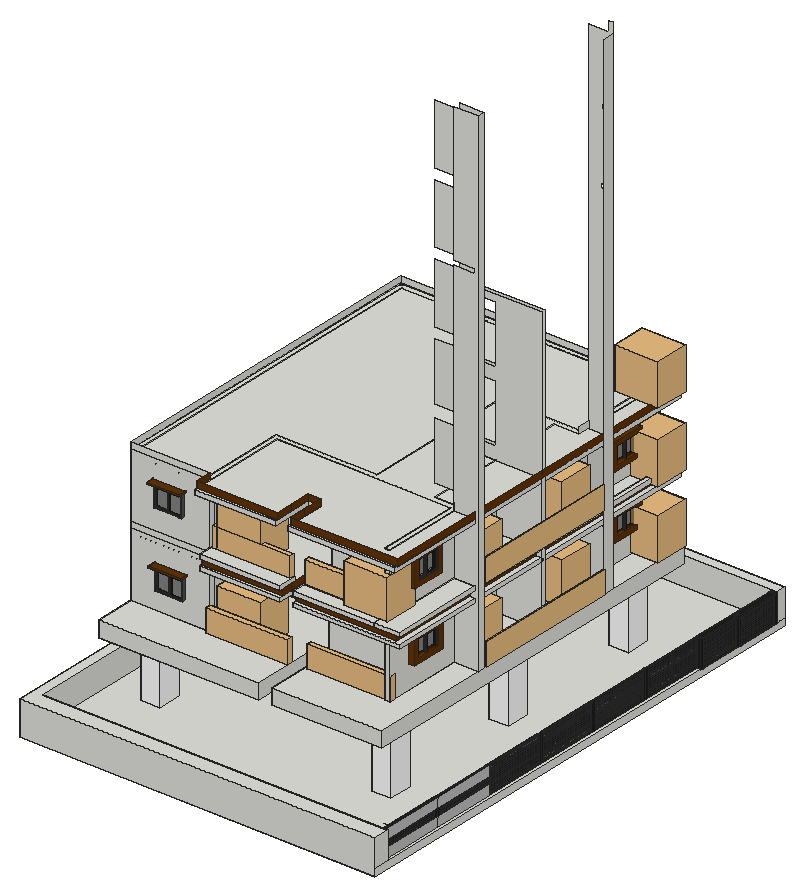
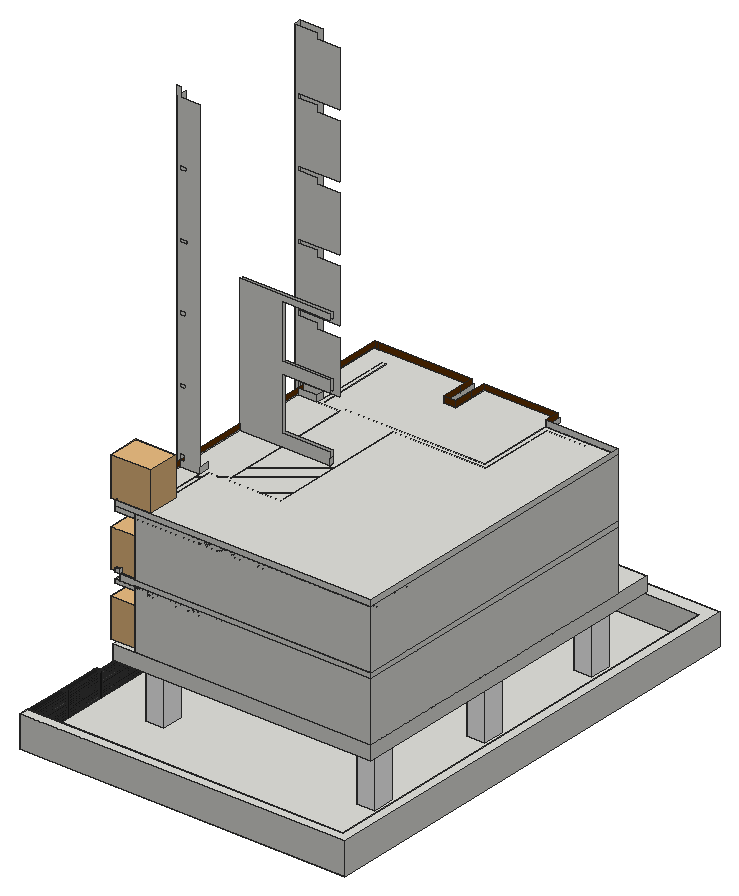
# SketchUp Ruby script. Lengths in inches.
U = 1.inch
M = Sketchup.active_model
def pt(a) = Geom::Point3d.new(a.map { |v| v * U })
def face(e, loops, mat)
  f = e.add_face(loops[0].map { |a| pt(a) })
  loops[1..].each { |l| e.add_face(l.map { |a| pt(a) }).erase! }
  f.material = f.back_material = mat if mat
  f
end
# faces: each face lists its corners as indices into pts; further lists are holes
def faces(e, pts, list, mat = nil) = list.each { |f| face(e, (f[0].is_a?(Array) ? f : [f]).map { |l| l.map { |i| pts[i] } }, mat) }
# xy, xz, yz: faces in a plane at the given z, y or x. An outline is a flat list of corners, or four numbers for a rectangle; further outlines are holes
def ring(l) = l.size == 4 ? [[l[0], l[1]], [l[2], l[1]], [l[2], l[3]], [l[0], l[3]]] : l.each_slice(2).to_a
def flat(e, list, mat, &to3) = list.each { |f| face(e, (f[0].is_a?(Array) ? f : [f]).map { |l| ring(l).map { |u, v| to3.(u, v) } }, mat) }
def xy(e, z, list, mat = nil) = flat(e, list, mat) { |x, y| [x, y, z] }
def xz(e, y, list, mat = nil) = flat(e, list, mat) { |x, z| [x, y, z] }
def yz(e, x, list, mat = nil) = flat(e, list, mat) { |y, z| [x, y, z] }
def lines(e, pts, list) = list.each { |a, b| e.add_line(pt(pts[a]), pt(pts[b])) }
# prism: a flat outline (further loops are holes) pulled along v
def prism(e, loops, v, mat = nil)
  f = face(e, loops, mat); d = Geom::Vector3d.new(v.map { |x| x * U })
  f.pushpull(f.normal.samedirection?(d) ? d.length : -d.length)
end
def box(e, o, s, mat = nil) = prism(e, [[o, [o[0] + s[0], o[1], o[2]], [o[0] + s[0], o[1] + s[1], o[2]], [o[0], o[1] + s[1], o[2]]]], [0, 0, s[2]], mat)
def at(x, y, z, deg = 0) = Geom::Transformation.translation(pt([x, y, z])) * Geom::Transformation.rotation(ORIGIN, Z_AXIS, deg.degrees)
def axes(o, x, y, z) = Geom::Transformation.new([*x, 0, *y, 0, *z, 0, *pt(o).to_a, 1])
def part(name) = M.definitions.add(name)
# library, detail: a bought-in or finely detailed component or shape, given as its bounding box
def library(name, o, s) = part(name).tap { |d| box(d.entities, o, s) }
def detail(e, o, s) = box(e.add_group.entities, o, s)
def put(e, d, t, mat = nil) = e.add_instance(d, t).tap { |i| i.material = mat if mat }
def group(e, t, mat = nil) = e.add_group.tap { |g| g.transformation = t; g.material = mat if mat }.entities
root = M.entities
M.materials.add("Color_008").color = [30, 30, 30]
M.materials.add("Glass_Tinted_Gray").color = [0, 0, 0]
M.materials["Glass_Tinted_Gray"].alpha = 0.125
M.materials.add("[0055_LightGoldenrodYellow]").color = [250, 250, 210]
M.materials.add("[0131_Silver]").color = [192, 192, 192]
M.materials.add("[0134_DimGray]").color = [105, 105, 105]
M.materials.add("[0135_DarkGray]").color = [81, 81, 81]
M.materials.add("[Color C08]").color = [102, 51, 0]
M.materials.add("[Color M00]").color = [255, 255, 255]
M.materials.add("[Mirror 02]").color = [229, 229, 229]
M.materials.add("[Terrazzo Light Blue]").color = [196, 214, 227]
c1 = part("Gate infill panel")
box(c1.entities,[0,0,-9.84],[39.64,0.39,36.58])
c2 = part("Gate frame stile")
box(c2.entities,[0,0,0],[1.9,0.97,93.54])
c3 = part("Gate slat \#1")
box(c3.entities,[2.95,0,-2.03],[0.99,0.97,40.94])
c4 = part("Gate slat")
box(c4.entities,[0,0,-2.03],[1.97,0.97,40.94])
c5 = part("Slatted gate leaf")
p = [[42.85,0.97,43.31],[42.85,0.97,44.29]]
lines(c5.entities,p,[[0,1]])
put(c5.entities,c2,axes([87.6,0,0],[1,0,0],[0,1,0],[0,0,0.92593]),"Color_008")
put(c5.entities,c2,axes([0,0,0],[1,0,0],[0,1,0],[0,0,0.92593]),"Color_008")
put(c5.entities,c2,axes([42.85,0,0],[1,0,0],[0,1,0],[0,0,0.92593]),"Color_008")
put(c5.entities,c2,axes([44.75,0,0],[1,0,0],[0,1,0],[0,0,0.92593]),"Color_008")
put(c5.entities,c3,axes([3.9375,0,6.89],[0,0,-1],[0,1,0],[1,0,0]),"[0134_DimGray]")
put(c5.entities,c3,axes([48.6875,0,6.89],[0,0,-1],[0,1,0],[1,0,0]),"[0134_DimGray]")
put(c5.entities,c3,axes([48.6875,0,11.71],[0,0,-1],[0,1,0],[1,0,0]),"[0134_DimGray]")
put(c5.entities,c4,axes([48.6875,0,6.79],[0,0,-1],[0,1,0],[1,0,0]),"Color_008")
put(c5.entities,c4,axes([3.9375,0,6.79],[0,0,-1],[0,1,0],[1,0,0]),"Color_008")
put(c5.entities,c3,axes([3.9375,0,11.71],[0,0,-1],[0,1,0],[1,0,0]),"[0134_DimGray]")
put(c5.entities,c4,axes([3.9375,0,11.61],[0,0,-1],[0,1,0],[1,0,0]),"Color_008")
put(c5.entities,c3,axes([3.9375,0,16.54],[0,0,-1],[0,1,0],[1,0,0]),"[0134_DimGray]")
put(c5.entities,c3,axes([48.6875,0,16.54],[0,0,-1],[0,1,0],[1,0,0]),"[0134_DimGray]")
put(c5.entities,c3,axes([48.6875,0,21.36],[0,0,-1],[0,1,0],[1,0,0]),"[0134_DimGray]")
put(c5.entities,c4,axes([48.6875,0,11.61],[0,0,-1],[0,1,0],[1,0,0]),"Color_008")
put(c5.entities,c3,axes([3.9375,0,21.36],[0,0,-1],[0,1,0],[1,0,0]),"[0134_DimGray]")
put(c5.entities,c4,axes([3.9375,0,26.08],[0,0,-1],[0,1,0],[1,0,0]),"Color_008")
put(c5.entities,c3,axes([3.9375,0,31],[0,0,-1],[0,1,0],[1,0,0]),"[0134_DimGray]")
put(c5.entities,c3,axes([3.9375,0,26.18],[0,0,-1],[0,1,0],[1,0,0]),"[0134_DimGray]")
put(c5.entities,c4,axes([48.6875,0,30.91],[0,0,-1],[0,1,0],[1,0,0]),"Color_008")
put(c5.entities,c4,axes([48.6875,0,21.26],[0,0,-1],[0,1,0],[1,0,0]),"Color_008")
put(c5.entities,c4,axes([3.9375,0,21.26],[0,0,-1],[0,1,0],[1,0,0]),"Color_008")
put(c5.entities,c4,axes([48.6875,0,41.7],[0,0,-1],[0,1,0],[1,0,0]),"Color_008")
put(c5.entities,c4,axes([48.6875,0,26.08],[0,0,-1],[0,1,0],[1,0,0]),"Color_008")
put(c5.entities,c4,axes([3.9375,0,35.73],[0,0,-1],[0,1,0],[1,0,0]),"Color_008")
put(c5.entities,c4,axes([3.9375,0,41.7],[0,0,-1],[0,1,0],[1,0,0]),"Color_008")
put(c5.entities,c4,axes([48.6875,0,35.73],[0,0,-1],[0,1,0],[1,0,0]),"Color_008")
put(c5.entities,c3,axes([48.6875,0,31],[0,0,-1],[0,1,0],[1,0,0]),"[0134_DimGray]")
put(c5.entities,c3,axes([48.6875,0,26.18],[0,0,-1],[0,1,0],[1,0,0]),"[0134_DimGray]")
put(c5.entities,c3,axes([3.9375,0,67.42],[0,0,-1],[0,1,0],[1,0,0]),"[0134_DimGray]")
put(c5.entities,c4,axes([48.6875,0,57.68],[0,0,-1],[0,1,0],[1,0,0]),"Color_008")
put(c5.entities,c4,axes([48.6875,0,52.85],[0,0,-1],[0,1,0],[1,0,0]),"Color_008")
put(c5.entities,c4,axes([3.9375,0,30.91],[0,0,-1],[0,1,0],[1,0,0]),"Color_008")
put(c5.entities,c3,axes([48.6875,0,57.78],[0,0,-1],[0,1,0],[1,0,0]),"[0134_DimGray]")
put(c5.entities,c4,axes([48.6875,0,62.5],[0,0,-1],[0,1,0],[1,0,0]),"Color_008")
put(c5.entities,c4,axes([3.9375,0,57.68],[0,0,-1],[0,1,0],[1,0,0]),"Color_008")
put(c5.entities,c4,axes([3.9375,0,62.5],[0,0,-1],[0,1,0],[1,0,0]),"Color_008")
put(c5.entities,c3,axes([48.6875,0,67.42],[0,0,-1],[0,1,0],[1,0,0]),"[0134_DimGray]")
put(c5.entities,c3,axes([48.6875,0,62.6],[0,0,-1],[0,1,0],[1,0,0]),"[0134_DimGray]")
put(c5.entities,c3,axes([3.9375,0,62.6],[0,0,-1],[0,1,0],[1,0,0]),"[0134_DimGray]")
put(c5.entities,c4,axes([48.6875,0,46.88],[0,0,-1],[0,1,0],[1,0,0]),"Color_008")
put(c5.entities,c4,axes([3.9375,0,52.85],[0,0,-1],[0,1,0],[1,0,0]),"Color_008")
put(c5.entities,c4,axes([3.9375,0,46.88],[0,0,-1],[0,1,0],[1,0,0]),"Color_008")
put(c5.entities,c3,axes([3.9375,0,57.78],[0,0,-1],[0,1,0],[1,0,0]),"[0134_DimGray]")
put(c5.entities,c4,axes([48.6875,0,16.4375],[0,0,-1],[0,1,0],[1,0,0]),"Color_008")
put(c5.entities,c4,axes([3.9375,0,16.4375],[0,0,-1],[0,1,0],[1,0,0]),"Color_008")
put(c5.entities,c4,axes([48.6875,0,1.97],[0,0,-1],[0,1,0],[1,0,0]),"Color_008")
put(c5.entities,c4,axes([3.9375,0,1.97],[0,0,-1],[0,1,0],[1,0,0]),"Color_008")
put(c5.entities,c3,axes([3.9375,0,81.89],[0,0,-1],[0,1,0],[1,0,0]),"[0134_DimGray]")
put(c5.entities,c4,axes([48.6875,0,72.15],[0,0,-1],[0,1,0],[1,0,0]),"Color_008")
put(c5.entities,c4,axes([48.6875,0,67.32],[0,0,-1],[0,1,0],[1,0,0]),"Color_008")
put(c5.entities,c3,axes([48.6875,0,72.24],[0,0,-1],[0,1,0],[1,0,0]),"[0134_DimGray]")
put(c5.entities,c3,axes([3.9375,0,72.24],[0,0,-1],[0,1,0],[1,0,0]),"[0134_DimGray]")
put(c5.entities,c4,axes([3.9375,0,72.15],[0,0,-1],[0,1,0],[1,0,0]),"Color_008")
put(c5.entities,c3,axes([3.9375,0,77.07],[0,0,-1],[0,1,0],[1,0,0]),"[0134_DimGray]")
put(c5.entities,c3,axes([48.6875,0,81.89],[0,0,-1],[0,1,0],[1,0,0]),"[0134_DimGray]")
put(c5.entities,c4,axes([3.9375,0,76.97],[0,0,-1],[0,1,0],[1,0,0]),"Color_008")
put(c5.entities,c4,axes([48.6875,0,76.97],[0,0,-1],[0,1,0],[1,0,0]),"Color_008")
put(c5.entities,c3,axes([48.6875,0,77.07],[0,0,-1],[0,1,0],[1,0,0]),"[0134_DimGray]")
put(c5.entities,c4,axes([3.9375,0,67.32],[0,0,-1],[0,1,0],[1,0,0]),"Color_008")
put(c5.entities,c4,axes([48.6875,0,86.61],[0,0,-1],[0,1,0],[1,0,0]),"Color_008")
put(c5.entities,c4,axes([48.6875,0,81.79],[0,0,-1],[0,1,0],[1,0,0]),"Color_008")
put(c5.entities,c3,axes([3.9375,0,86.71],[0,0,-1],[0,1,0],[1,0,0]),"[0134_DimGray]")
put(c5.entities,c3,axes([48.6875,0,86.71],[0,0,-1],[0,1,0],[1,0,0]),"[0134_DimGray]")
put(c5.entities,c4,axes([3.9375,0,86.61],[0,0,-1],[0,1,0],[1,0,0]),"Color_008")
put(c5.entities,c4,axes([3.9375,0,81.79],[0,0,-1],[0,1,0],[1,0,0]),"Color_008")
put(c5.entities,c3,axes([48.6875,0,35.83],[0,0,-1],[0,1,0],[1,0,0]),"[0134_DimGray]")
put(c5.entities,c3,axes([3.9375,0,35.83],[0,0,-1],[0,1,0],[1,0,0]),"[0134_DimGray]")
c6 = part("Gate infill panel \#1")
box(c6.entities,[0,0,-1.97],[52.81,0.39,23.62])
c7 = part("Porton casa")
put(c7.entities,c1,axes([2026.52,648.38,306.58],[0,-3.00253,0],[2.8696,0,0],[0,0,0.48432]),"[0131_Silver]")
put(c7.entities,c1,axes([2026.52,767.39,338.47],[0,-3.00253,0],[2.8696,0,0],[0,0,0.48432]),"[0131_Silver]")
put(c7.entities,c5,axes([2023.74,772.67,300.63],[0,-2.77742,0],[2.8696,0,0],[0,0,0.6]),"[0055_LightGoldenrodYellow]")
put(c7.entities,c1,axes([2026.52,767.39,306.58],[0,-3.00253,0],[2.8696,0,0],[0,0,0.48432]),"[0131_Silver]")
put(c7.entities,c6,axes([2022.61,772.67,320.71],[0,-2.3537,0],[2.8696,0,0],[0,0,0.6]),"Color_008")
put(c7.entities,c1,axes([2026.52,648.38,338.47],[0,-3.00253,0],[2.8696,0,0],[0,0,0.48432]),"[0131_Silver]")
put(c7.entities,c6,axes([2022.61,648.38,320.71],[0,-2.3537,0],[2.8696,0,0],[0,0,0.6]),"Color_008")
put(c7.entities,c5,axes([2023.74,1012.92,300.63],[0,-2.77742,0],[2.8696,0,0],[0,0,0.6]),"[0055_LightGoldenrodYellow]")
put(c7.entities,c5,axes([2023.74,1256.22,300.63],[0,-2.77742,0],[2.8696,0,0],[0,0,0.6]),"[0055_LightGoldenrodYellow]")
put(c7.entities,c5,axes([2023.74,1426.375,300.63],[0,-1.96025,0],[10.8312,0,0],[0,0,0.6]),"[0055_LightGoldenrodYellow]")
c8 = part("Group\#10")
box(c8.entities,[49.375,41.9375,0],[35.875,43.3125,120],"[Color M00]")
c9 = library("Wagner Glass Railing",[9.08,102.375,1.53],[2.51,145.5,42.05])
c10 = library("Round Planter with Plant",[-35.48,-39.77,0],[80.62,63.55,77.875])
c11 = part("PENTEK_RP Fineline 50S_Sliding_DoorCase_E1")
box(c11.entities,[0,0,0],[1.51,3.66,99.27],"[0135_DarkGray]")
c12 = part("PENTEK_RP Fineline 50S_SlidingDooe_Case_E2")
box(c12.entities,[0,0,0],[96.25,3.66,1.51],"[0135_DarkGray]")
c13 = part("pentek_RP Fineline 50S_SlidingDoor_Case")
put(c13.entities,c11,at(97.76,0,0))
put(c13.entities,c12,at(1.51,0,0))
put(c13.entities,c11,at(0,0,0))
put(c13.entities,c12,at(1.51,0,97.76))
c14 = part("PENTEK_RP Fineline 50S_SlidingDoor_GlazingBead_2")
box(c14.entities,[0,0,0],[0.56,0.59,94.39],"[0135_DarkGray]")
c15 = part("PENTEK_RP Fineline 50S_SlidingDoor_Glass")
box(c15.entities,[0,0,0],[46.58,0.16,94.39],"Glass_Tinted_Gray")
c16 = part("PENTEK_RP Fineline 50S_SlidingDoor_GlazingBead")
box(c16.entities,[0,0,0],[45.47,0.59,0.56],"[0135_DarkGray]")
c17 = part("PENTEK_RP Fineline 50S_SlidingDoor_Leaf_E1")
xy(c17.entities,0,[[0,0,0.93,1.97],[0.93,1.57,1.49,1.97]],"[0135_DarkGray]")
xy(c17.entities,96.25,[[0,0,0.93,0,0.93,1.57,1.49,1.57,1.49,1.97,0,1.97]],"[0135_DarkGray]")
xz(c17.entities,0,[[0,0,0.93,96.25]],"[0135_DarkGray]")
xz(c17.entities,1.57,[[0.93,0,1.49,95.32],[0.93,95.32,1.49,96.25]],"[0135_DarkGray]")
xz(c17.entities,1.97,[[0,0,1.49,96.25]],"[0135_DarkGray]")
yz(c17.entities,0,[[0,0,1.97,96.25]],"[0135_DarkGray]")
yz(c17.entities,0.93,[[0,0,1.57,0.93],[0,0.93,1.57,95.32],[0,95.32,1.57,96.25]],"[0135_DarkGray]")
yz(c17.entities,1.49,[[1.57,0,1.97,95.32],[1.57,95.32,1.97,96.25]],"[0135_DarkGray]")
c18 = part("PENTEK_RP Fineline 50S_SlidingDoor_Leaf_E2")
xy(c18.entities,0,[[0,0,0,1.57,0.56,1.57,0.56,1.97,46.02,1.97,46.02,1.57,46.58,1.57,46.58,0]],"[0135_DarkGray]")
xy(c18.entities,0.93,[[0,0,46.58,1.57]],"[0135_DarkGray]")
xy(c18.entities,1.49,[[0.56,1.57,46.02,1.97]],"[0135_DarkGray]")
xz(c18.entities,0,[[0,0,46.58,0.93]],"[0135_DarkGray]")
xz(c18.entities,1.57,[[0,0,0.56,0.93],[46.02,0,46.58,0.93],[0.56,0.93,46.02,1.49]],"[0135_DarkGray]")
xz(c18.entities,1.97,[[0.56,0,46.02,1.49]],"[0135_DarkGray]")
yz(c18.entities,0,[[0,0,1.57,0.93]],"[0135_DarkGray]")
yz(c18.entities,0.56,[[1.57,0,1.97,0.93],[1.57,0.93,1.97,1.49]],"[0135_DarkGray]")
yz(c18.entities,46.02,[[1.57,0,1.97,0.93],[1.57,0.93,1.97,1.49]],"[0135_DarkGray]")
yz(c18.entities,46.58,[[0,0,1.57,0.93]],"[0135_DarkGray]")
c19 = part("PENTEK_RP Fineline S_SlidingDoor_Leaf1")
put(c19.entities,c14,at(0.93,0,0.93))
put(c19.entities,c14,at(46.96,0,0.93))
put(c19.entities,c15,at(1.49,1.42,0.93))
put(c19.entities,c16,at(1.49,0,0.93))
put(c19.entities,c15,at(1.49,0.59,0.93),"[Terrazzo Light Blue]")
put(c19.entities,c17,at(0,0,0))
put(c19.entities,c17,axes([48.44,0,0],[-1,0,0],[0,1,0],[0,0,1]))
put(c19.entities,c18,axes([0.93,0,96.25],[1,0,0],[0,1,0],[0,0,-1]))
put(c19.entities,c18,at(0.93,0,0))
put(c19.entities,c16,at(1.49,0,94.77))
c20 = part("PENTEK_RP Fineline 50S_SlidingDoor_Leaf2")
put(c20.entities,c15,at(1.49,1.42,0.93))
put(c20.entities,c16,at(1.49,0,94.77))
put(c20.entities,c14,at(46.96,0,0.93))
put(c20.entities,c15,at(1.49,0.59,0.93),"[Mirror 02]")
put(c20.entities,c14,at(0.93,0,0.93))
put(c20.entities,c17,at(0,0,0))
put(c20.entities,c17,axes([48.44,0,0],[-1,0,0],[0,1,0],[0,0,1]))
put(c20.entities,c16,at(1.49,0,0.93))
put(c20.entities,c18,axes([0.93,0,96.25],[1,0,0],[0,1,0],[0,0,-1]))
put(c20.entities,c18,at(0.93,0,0))
c21 = part("PENTEK - Slimmest Steel Sliding Door / Window\#1")
put(c21.entities,c13,at(0,-1.88,-0.09))
put(c21.entities,c19,at(1.51,-2.27,1.42))
put(c21.entities,c20,at(49.32,-0.3,1.42))
c22 = part("Group\#9")
box(c22.entities,[0,0,0],[60.1875,3.0625,15.3125])
xy(root,-162.0625,[[0,0,659.75,950.625]])
xy(root,-149.5,[[19.4375,28.625,659.75,931.79]])
xy(root,-98,[[0,0,659.75,0,659.75,28.625,19.4375,28.625,19.4375,931.79,659.75,931.79,659.75,950.625,0,950.625]])
xy(root,0,[[53.0625,117.84,350.31,117.84,350.31,232.22,374.31,232.22,374.31,117.84,577.93,117.84,577.93,191.22,578.3125,191.22,578.3125,341.375,533.0625,341.375,533.0625,191.22,524.0625,191.22,524.0625,241.82,381.04,241.82,381.04,346.01,200.56,346.01,200.56,191.22,53.0625,191.22],[53.0625,191.22,200.56,191.22,200.56,346.01,381.04,346.01,381.04,241.82,524.0625,241.82,524.0625,192.09,533.0625,192.09,533.0625,355.01,486.8125,355.01,486.8125,495.28,388.3125,495.28,388.3125,502.74,486.8125,502.74,486.8125,631.35,533.0625,631.35,533.0625,638.86,524.0625,640.35,379.3125,640.35,379.3125,355.01,191.56,355.01,191.56,200.22,62.0625,200.22,62.0625,809.84,524.0625,809.84,524.0625,640.35,533.0625,638.86,533.0625,818.16,53.0625,818.16],[524.0625,191.22,533.0625,192.09],[62.0625,200.22,191.56,200.22,191.56,355.01,379.3125,355.01,379.3125,640.35,524.0625,640.35,524.0625,809.84,62.0625,809.84],[486.8125,355.01,578.3125,495.28],
  [572.25,495.28,578.3125,502.74],[486.8125,502.74,578.3125,631.35],[533.0625,631.35,578.3125,631.35,533.0625,638.86],[578.3125,631.35,578.3125,653.47,533.0625,653.47,533.0625,638.86],[533.0625,653.47,578.3125,818.16]])
xy(root,44.43,[[533.0625,234.1,545.1875,299.28],[533.0625,696.28,545.1875,761.47]],"[Color C08]")
xy(root,52.48,[[533.0625,242.15,545.1875,291.23],[533.0625,704.34,545.1875,753.42]],"[Color C08]")
xy(root,85.5625,[[533.0625,242.15,545.1875,291.23],[533.0625,704.34,545.1875,753.42]])
xy(root,93.62,[[533.0625,234.1,545.1875,299.28],[533.0625,696.28,545.1875,761.47]],"[Color C08]")
xy(root,112.625,[[381.04,241.82,524.0625,346.01]])
xy(root,120,[[[53.0625,191.22,200.56,191.22,200.56,346.01,524.0625,346.01,524.0625,191.22,533.0625,191.22,533.0625,355.01,486.8125,355.01,486.8125,495.28,388.3125,495.28,388.3125,502.74,486.8125,502.74,486.8125,631.35,533.0625,631.35,533.0625,818.16,53.0625,818.16],[62.0625,200.22,62.0625,809.84,524.0625,809.84,524.0625,640.35,379.3125,640.35,379.3125,355.01,191.56,355.01,191.56,200.22]]])
xy(root,132,[[200.56,165.97,350.31,191.22],[374.31,165.97,524.0625,191.22],[524.25,165.97,524.25,191.22,533.0625,191.22,533.0625,341.375,572.25,341.375,572.25,165.97],[[53.0625,191.22,200.56,191.22,200.56,346.01,389.59,346.01,389.59,237.76,524.0625,237.76,524.0625,191.22,533.0625,191.22,533.0625,355.01,486.8125,355.01,486.8125,495.28,388.3125,495.28,388.3125,502.74,486.8125,502.74,486.8125,631.35,533.0625,631.35,533.0625,818.16,53.0625,818.16],[62.0625,200.22,62.0625,809.84,524.0625,809.84,524.0625,640.35,379.3125,640.35,379.3125,355.01,191.56,355.01,191.56,200.22]],[62.0625,200.22,191.56,200.22,191.56,355.01,379.3125,355.01,379.3125,640.35,524.0625,640.35,524.0625,809.84,62.0625,809.84],
  [200.56,200.22,350.31,200.22,350.31,232.22,374.31,232.22,374.31,200.22,524.0625,200.22,524.0625,237.76,389.59,237.76,389.59,346.01,200.56,346.01],[486.8125,355.01,560.01,355.01,560.01,631.35,486.8125,631.35,486.8125,502.74,388.3125,502.74,388.3125,495.28,486.8125,495.28],[533.0625,641.54,572.25,641.54,572.25,653.47,563.82,653.47,563.82,818.16,533.0625,818.16]])
xy(root,139.375,[[200.56,165.97,350.31,200.22],[374.31,165.97,524.0625,200.22]])
xy(root,139.6875,[[524.25,165.97,572.25,165.97,572.25,341.375,533.0625,341.375,533.0625,191.22,524.25,191.22]])
xy(root,140.1875,[[560.01,355.01,572.25,631.35],[563.82,653.47,572.25,818.16]])
xy(root,163.74,[[533.0625,696.28,545.1875,761.47]],"[Color C08]")
xy(root,171.8,[[533.0625,704.34,545.1875,753.42]],"[Color C08]")
xy(root,171.99,[[533.0625,236.27,545.1875,298.83]],"[Color C08]")
xy(root,180.05,[[533.0625,244.32,545.1875,290.77]])
xy(root,204.875,[[533.0625,704.34,545.1875,753.42]])
xy(root,212.93,[[533.0625,696.28,545.1875,761.47]],"[Color C08]")
xy(root,217.25,[[533.0625,244.32,545.1875,290.77]],"[Color C08]")
xy(root,225.3,[[533.0625,236.27,545.1875,298.83]],"[Color C08]")
xy(root,243.8125,[[389.59,237.76,524.0625,346.01]])
xy(root,252,[[562.5625,155.07,572.25,162],[[53.0625,191.22,200.56,191.22,200.56,346.01,524.0625,346.01,524.0625,191.22,533.0625,191.22,533.0625,355.01,486.8125,355.01,486.8125,495.28,388.3125,495.28,388.3125,502.74,486.8125,502.74,486.8125,631.35,533.0625,631.35,533.0625,818.16,53.0625,818.16],[62.0625,200.22,62.0625,809.84,524.0625,809.84,524.0625,640.35,379.3125,640.35,379.3125,355.01,191.56,355.01,191.56,200.22]]])
xz(root,0,[[0,-162.0625,659.75,-98]])
xz(root,28.625,[[19.4375,-149.5,659.75,-98]])
xz(root,165.97,[[200.56,132,350.31,139.375],[374.31,132,524.0625,139.375],[524.25,132,572.25,139.6875]])
xz(root,191.22,[[53.0625,0,200.56,120],[524.0625,0,533.0625,120],[53.0625,132,200.56,252],[374.31,132,524.0625,139.375],[524.0625,132,524.25,132,524.25,139.6875,533.0625,139.6875,533.0625,252,524.0625,252],
  [524.25,132,533.0625,139.6875]])
xz(root,200.22,[[62.0625,0,191.56,120],[62.0625,132,191.56,252],[200.56,132,350.31,139.375],[374.31,132,524.0625,139.375]])
xz(root,234.1,[[533.0625,44.43,545.1875,93.62]],"[Color C08]")
xz(root,236.27,[[533.0625,171.99,545.1875,225.3]],"[Color C08]")
xz(root,237.76,[[389.59,132,524.0625,243.8125]])
xz(root,241.82,[[381.04,0,524.0625,112.625]])
xz(root,242.15,[[533.0625,52.48,545.1875,85.5625]],"[Color C08]")
xz(root,244.32,[[533.0625,180.05,545.1875,217.25]],"[Color C08]")
xz(root,290.77,[[533.0625,180.05,545.1875,217.25]],"[Color C08]")
xz(root,291.23,[[533.0625,52.48,545.1875,85.5625]],"[Color C08]")
xz(root,298.83,[[533.0625,171.99,545.1875,225.3]],"[Color C08]")
xz(root,299.28,[[533.0625,44.43,545.1875,93.62]],"[Color C08]")
xz(root,341.375,[[533.0625,0,578.3125,0,578.3125,924,533.0625,924,533.0625,668.1875,572.25,668.1875,572.25,660,533.0625,660,533.0625,139.6875,572.25,139.6875,572.25,132,533.0625,132],[533.0625,132,572.25,139.6875]])
xz(root,346.01,[[200.56,0,381.04,0,381.04,112.625,524.0625,112.625,524.0625,120,200.56,120],[200.56,132,389.59,132,389.59,243.8125,524.0625,243.8125,524.0625,252,200.56,252]])
xz(root,355.01,[[191.56,0,379.3125,120],[486.8125,0,486.8125,120,533.0625,120,533.0625,132,486.8125,132,486.8125,252,533.0625,252,533.0625,264,572.25,264,572.25,276.5625,486.8125,276.5625,486.8125,384,533.0625,384,533.0625,396,572.25,396,572.25,407.125,486.8125,407.125,486.8125,516,533.0625,516,533.0625,528,572.25,528,572.25,535.4375,486.8125,535.4375,486.8125,648,533.0625,648,533.0625,660,572.25,660,572.25,668.1875,486.8125,668.1875,486.8125,780,533.0625,780,533.0625,792,572.25,792,572.25,800.1875,486.8125,800.1875,486.8125,912,533.0625,912,533.0625,924,578.3125,924,578.3125,0],[191.56,132,379.3125,252],[560.01,132,572.25,140.1875]])
xz(root,495.28,[[388.3125,0,486.8125,120],[486.8125,0,572.25,0,572.25,528,388.3125,528,388.3125,516,486.8125,516,486.8125,407.125,388.3125,407.125,388.3125,384,486.8125,384,486.8125,276.5625,388.3125,276.5625,388.3125,252,486.8125,252,486.8125,132,388.3125,132,388.3125,120,486.8125,120],[388.3125,132,486.8125,252]])
xz(root,502.74,[[388.3125,0,486.8125,120],[486.8125,0,486.8125,120,388.3125,120,388.3125,132,486.8125,132,486.8125,252,388.3125,252,388.3125,276.5625,486.8125,276.5625,486.8125,384,388.3125,384,388.3125,407.125,486.8125,407.125,486.8125,516,388.3125,516,388.3125,528,572.25,528,572.25,0],[388.3125,132,486.8125,252]])
xz(root,631.35,[[560.01,132,572.25,140.1875]])
xz(root,640.35,[[379.3125,0,524.0625,120],[379.3125,132,524.0625,252]])
xz(root,653.47,[[[533.0625,0,578.3125,0,578.3125,943.375,570.58,943.375,570.58,924,533.0625,924],[555.82,660,572.25,668.1875],[562.82,264,572.25,276.5625],[557.85,792,572.25,800.1875],[559.99,396,572.25,404.1875],[561.5,528,572.25,536.1875],[563.82,132,572.25,140.1875]],[563.82,132,572.25,140.1875]])
xz(root,696.28,[[533.0625,44.43,545.1875,93.62],[533.0625,163.74,545.1875,212.93]],"[Color C08]")
xz(root,704.34,[[533.0625,52.48,545.1875,85.5625],[533.0625,171.8,545.1875,204.875]],"[Color C08]")
xz(root,753.42,[[533.0625,52.48,545.1875,85.5625],[533.0625,171.8,545.1875,204.875]],"[Color C08]")
xz(root,761.47,[[533.0625,44.43,545.1875,93.62],[533.0625,163.74,545.1875,212.93]],"[Color C08]")
xz(root,809.84,[[62.0625,0,524.0625,120],[62.0625,132,524.0625,252]])
xz(root,818.16,[[53.0625,0,533.0625,120],[53.0625,132,533.0625,252],[563.82,132,572.25,140.1875]])
xz(root,931.79,[[19.4375,-149.5,659.75,-98]])
xz(root,950.625,[[0,-162.0625,659.75,-98]])
yz(root,0,[[0,-162.0625,950.625,-98]])
yz(root,19.4375,[[28.625,-149.5,931.79,-98]])
yz(root,53.0625,[[191.22,0,818.16,120],[191.22,132,818.16,252]])
yz(root,62.0625,[[200.22,0,809.84,120],[200.22,132,809.84,252]])
yz(root,191.56,[[200.22,0,355.01,120],[200.22,132,355.01,252]])
yz(root,200.56,[[191.22,0,200.22,120],[200.22,0,346.01,120],[165.97,132,191.22,139.375],[191.22,132,200.22,139.375],[200.22,132,346.01,252],
  [191.22,139.375,200.22,252]])
yz(root,350.31,[[165.97,132,200.22,139.375]])
yz(root,374.31,[[165.97,132,191.22,139.375],[191.22,132,200.22,139.375]])
yz(root,379.3125,[[355.01,0,640.35,120],[355.01,132,640.35,252]])
yz(root,381.04,[[241.82,0,346.01,112.625]])
yz(root,388.3125,[[495.28,0,502.74,120],[495.28,120,502.74,132],[495.28,132,502.74,252],[495.28,252,502.74,264]])
yz(root,389.59,[[237.76,132,346.01,243.8125]])
yz(root,486.8125,[[355.01,0,495.28,120],[502.74,0,631.35,120],[355.01,132,495.28,252],[502.74,132,631.35,252]])
yz(root,524.0625,[[191.22,0,200.22,120],[200.22,0,200.22,120,346.01,120,346.01,112.625,241.82,112.625,241.82,0],[640.35,0,809.84,120],[165.97,132,191.22,139.375],[191.22,132,200.22,139.375],
  [200.22,132,200.22,252,346.01,252,346.01,243.8125,237.76,243.8125,237.76,132],[640.35,132,809.84,252],[191.22,139.375,200.22,252]])
yz(root,524.25,[[165.97,132,191.22,139.6875]])
yz(root,533.0625,[[[191.22,0,341.375,120],[234.1,44.43,299.28,93.62]],[[653.47,0,818.16,120],[696.28,44.43,761.47,93.62]],[242.15,52.48,291.23,85.5625],[704.34,52.48,753.42,85.5625],[341.375,120,355.01,132],
  [631.35,120,653.47,132],[191.22,132,341.375,139.6875],[[653.47,132,818.16,252],[696.28,163.74,761.47,212.93]],[[191.22,139.6875,341.375,252],[236.27,171.99,298.83,225.3]],[704.34,171.8,753.42,204.875],
  [244.32,180.05,290.77,217.25],[341.375,252,355.01,264],[631.35,252,653.47,264]])
yz(root,545.1875,[[[234.1,44.43,299.28,93.62],[242.15,52.48,291.23,85.5625]],[[696.28,44.43,761.47,93.62],[704.34,52.48,753.42,85.5625]],[[696.28,163.74,761.47,212.93],[704.34,171.8,753.42,204.875]],[[236.27,171.99,298.83,225.3],[244.32,180.05,290.77,217.25]]],"[Color C08]")
yz(root,560.01,[[355.01,132,495.28,140.1875],[495.28,132,502.74,140.1875],[502.74,132,631.35,140.1875]])
yz(root,563.82,[[653.47,132,653.85,140.1875],[653.85,132,818.16,140.1875]])
yz(root,572.25,[[495.28,0,502.74,140.1875],[165.97,132,341.375,139.6875],[355.01,132,495.28,140.1875],[502.74,132,631.35,140.1875],[653.47,132,818.16,140.1875],
  [495.28,140.1875,502.74,252],[495.28,252,502.74,264]])
yz(root,578.3125,[[341.375,0,355.01,924],[631.35,0,653.47,924]])
yz(root,659.75,[[0,-162.0625,950.625,-149.5],[0,-149.5,28.625,-98],[931.79,-149.5,950.625,-98]])
p = [[524.0625,640.35,0],[533.0625,638.86,0],[578.3125,631.35,0],[578.3125,631.35,112.625],[524.0625,640.35,112.625],[532.5625,651.375,136.93],
  [578.3125,631.35,136.93],[578.3125,631.35,243.8125],[532.5625,651.375,243.8125],[374.31,191.22,132],[374.31,191.22,120],[350.31,191.22,132],
  [350.31,191.22,120],[374.31,191.22,264],[374.31,191.22,252],[350.31,191.22,264],[350.31,191.22,252],[577.93,191.22,0],
  [577.93,192.09,0],[200.56,191.22,264],[200.56,191.22,252],[572.25,341.375,252],[572.25,341.375,264],[562.5625,162,264],
  [562.5625,162,252],[572.25,162,252],[655.46,37.85,-95.375],[645.27,37.85,-95.375]]
faces(root,p,[[0,1,2,3,4],[5,6,7,8]])
lines(root,p,[[9,10],[11,12],[13,14],[15,16],[17,18],[19,20],[21,22],[23,24],[25,21],[26,27]])
put(root,c7,at(-1374.48,-494.58,-452.1))
g1 = group(root,at(53.0625,818.16,-12))
xy(g1,-17.5,[[0,-700.3125,0,0,525.25,0,525.25,-700.3125,321.25,-700.3125,321.25,-586.6875,297.25,-586.6875,297.25,-700.3125]],"[Color M00]")
xz(g1,-700.3125,[[0,-17.5,297.25,12],[321.25,-17.5,525.25,12]])
xz(g1,-586.6875,[[297.25,-17.5,321.25,12]])
xz(g1,0,[[0,-17.5,525.25,12]])
yz(g1,0,[[-700.3125,-17.5,0,12]])
yz(g1,297.25,[[-700.3125,-17.5,-586.6875,12]])
yz(g1,321.25,[[-700.3125,-17.5,-586.6875,12]])
yz(g1,525.25,[[-700.3125,-17.5,0,12]])
put(g1,c8,axes([114.88,-130.76,-17.5],[-1,0,0],[0,1,0],[0,0,-1]))
put(g1,c8,axes([114.88,-409.82,-17.5],[-1,0,0],[0,1,0],[0,0,-1]))
put(g1,c8,axes([114.88,-682.63,-17.5],[-1,0,0],[0,1,0],[0,0,-1]))
put(g1,c8,axes([543.06,-409.82,-17.5],[-1,0,0],[0,1,0],[0,0,-1]))
put(g1,c8,axes([543.06,-682.63,-17.5],[-1,0,0],[0,1,0],[0,0,-1]))
put(g1,c8,axes([543.06,-130.76,-17.5],[-1,0,0],[0,1,0],[0,0,-1]))
put(root,c9,axes([268.09,158.33,-3.19],[0,3.9,0],[1.07184,0,0],[0,0,1]))
put(root,c10,at(245.78,234.84,0))
put(root,c9,axes([569.23,165.24,-0.21],[1,0,0],[0,1.88042,0],[0,0,1]))
put(root,c9,axes([94.12,146.01,0.57],[0,3.9,0],[1.03969,0,0],[0,0,1]))
put(root,c10,at(540.42,789.45,4.14))
put(root,c10,at(515.72,394.78,5.34))
put(root,c10,at(515.28,598.17,5.9))
put(root,c21,axes([153.96,188.68,35.61],[-0.51717,0,0],[0,1.4209,0],[0,0,0.41395]))
put(root,c21,axes([538.58,292.4375,45.5625],[0,-0.51717,0],[-1.4209,0,0],[0,0,0.41395]))
put(root,c21,axes([538.58,754.625,45.5625],[0,-0.51717,0],[-1.4209,0,0],[0,0,0.41395]))
put(root,c22,axes([97.34,191.22,76.33],[1,0,0],[0,0,1],[0,-1,0]),"[Color C08]")
g2 = group(root,at(53.0625,818.16,120))
xy(g2,-7.375,[[147.5,-652.1875,147.5,-626.9375,0,-626.9375,0,0,519.1875,0,519.1875,-652.1875,321.25,-652.1875,321.25,-586.6875,297.25,-586.6875,297.25,-652.1875]])
xy(g2,0,[[147.5,-652.1875,297.25,-646.4375],[321.25,-652.1875,509.375,-646.4375],[509.375,-652.1875,519.1875,0],[147.5,-646.4375,297.25,-646.4375,297.25,-586.6875,321.25,-586.6875,321.25,-646.4375,509.375,-646.4375,509.375,0,0,0,0,-626.9375,147.5,-626.9375]])
xz(g2,-652.1875,[[147.5,-7.375,297.25,0],[321.25,-7.375,519.1875,0]])
xz(g2,-646.4375,[[147.5,0,297.25,12],[321.25,0,509.375,12]],"[Color C08]")
xz(g2,-626.9375,[[0,-7.375,147.5,0],[0,0,147.5,12]])
xz(g2,-586.6875,[[297.25,-7.375,321.25,0]])
xz(g2,-586.6875,[[297.25,0,321.25,12]],"[Color C08]")
xz(g2,0,[[0,-7.375,519.1875,0],[0,0,509.375,12]])
yz(g2,0,[[-626.9375,-7.375,0,0],[-626.9375,0,0,12]])
yz(g2,147.5,[[-652.1875,-7.375,-626.9375,0]])
yz(g2,147.5,[[-646.4375,0,-626.9375,12]],"[Color C08]")
yz(g2,297.25,[[-652.1875,-7.375,-586.6875,0]])
yz(g2,297.25,[[-646.4375,0,-586.6875,12]],"[Color C08]")
yz(g2,321.25,[[-652.1875,-7.375,-586.6875,0]])
yz(g2,321.25,[[-646.4375,0,-586.6875,12]],"[Color C08]")
yz(g2,509.375,[[-646.4375,0,0,12]],"[Color C08]")
yz(g2,519.1875,[[-652.1875,-7.375,0,0]])
put(root,c10,at(540.42,789.45,130.46))
put(root,c9,axes([79.84,158.33,131.74],[0,3.9,0],[1.07184,0,0],[0,0,1]))
put(root,c10,at(492.57,220.35,134.46))
put(root,c10,at(515.72,394.78,135.96))
put(root,c10,at(515.28,598.17,136.51))
put(root,c9,axes([271.66,155.82,137.83],[0,3.9,0],[1.01825,0,0],[0,0,1]))
put(root,c10,at(245.78,234.84,140.1875))
put(root,c9,axes([567.49,165.71,139.16],[1,0,0],[0,1.88042,0],[0,0,1]))
put(root,c21,axes([538.58,754.625,164.875],[0,-0.51717,0],[-1.4209,0,0],[0,0,0.41395]))
put(root,c21,axes([151.8125,188.68,173.23],[-0.51717,0,0],[0,1.4209,0],[0,0,0.41395]))
put(root,c21,axes([538.58,292.4375,178.5625],[0,-0.51717,0],[-1.4209,0,0],[0,0,0.41395]))
put(root,c22,axes([94.27,191.22,214.3],[1,0,0],[0,0,1],[0,-1,0]),"[Color C08]")
g3 = group(root,at(53.0625,818.16,252))
xy(g3,-8.1875,[[147.5,-663.09,147.5,-626.9375,0,-626.9375,0,0,519.1875,0,519.1875,-663.09,321.25,-663.09,321.25,-586.6875,297.25,-586.6875,297.25,-663.09]])
xy(g3,0,[[147.5,-663.09,297.25,-657.34],[321.25,-663.09,509.5,-657.34],[509.5,-663.09,519.1875,-657.34],[147.5,-657.34,297.25,-657.34,297.25,-586.6875,321.25,-586.6875,321.25,-657.34,519.1875,-657.34,519.1875,0,0,0,0,-626.9375,147.5,-626.9375]])
xz(g3,-663.09,[[147.5,-8.1875,297.25,0],[321.25,-8.1875,519.1875,0]])
xz(g3,-657.34,[[147.5,0,297.25,12],[321.25,0,519.1875,12]],"[Color C08]")
xz(g3,-626.9375,[[0,-8.1875,147.5,0],[0,0,147.5,12]])
xz(g3,-586.6875,[[297.25,-8.1875,321.25,0]])
xz(g3,-586.6875,[[297.25,0,321.25,12]],"[Color C08]")
xz(g3,0,[[0,-8.1875,519.1875,0],[0,0,519.1875,12]])
yz(g3,0,[[-626.9375,-8.1875,0,0],[-626.9375,0,0,12]])
yz(g3,147.5,[[-663.09,-8.1875,-626.9375,0]])
yz(g3,147.5,[[-657.34,0,-626.9375,12]],"[Color C08]")
yz(g3,297.25,[[-663.09,-8.1875,-586.6875,0]])
yz(g3,297.25,[[-657.34,0,-586.6875,12]],"[Color C08]")
yz(g3,321.25,[[-663.09,-8.1875,-586.6875,0]])
yz(g3,321.25,[[-657.34,0,-586.6875,12]],"[Color C08]")
yz(g3,519.1875,[[-663.09,-8.1875,0,0]])
yz(g3,519.1875,[[-657.34,0,0,12]],"[Color C08]")
put(root,c10,at(540.42,789.45,261.14))
